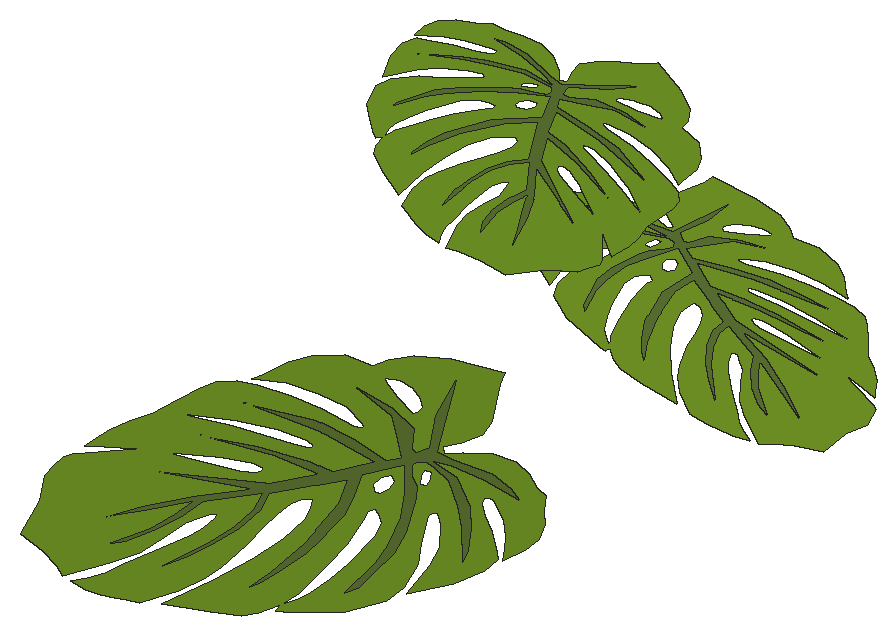
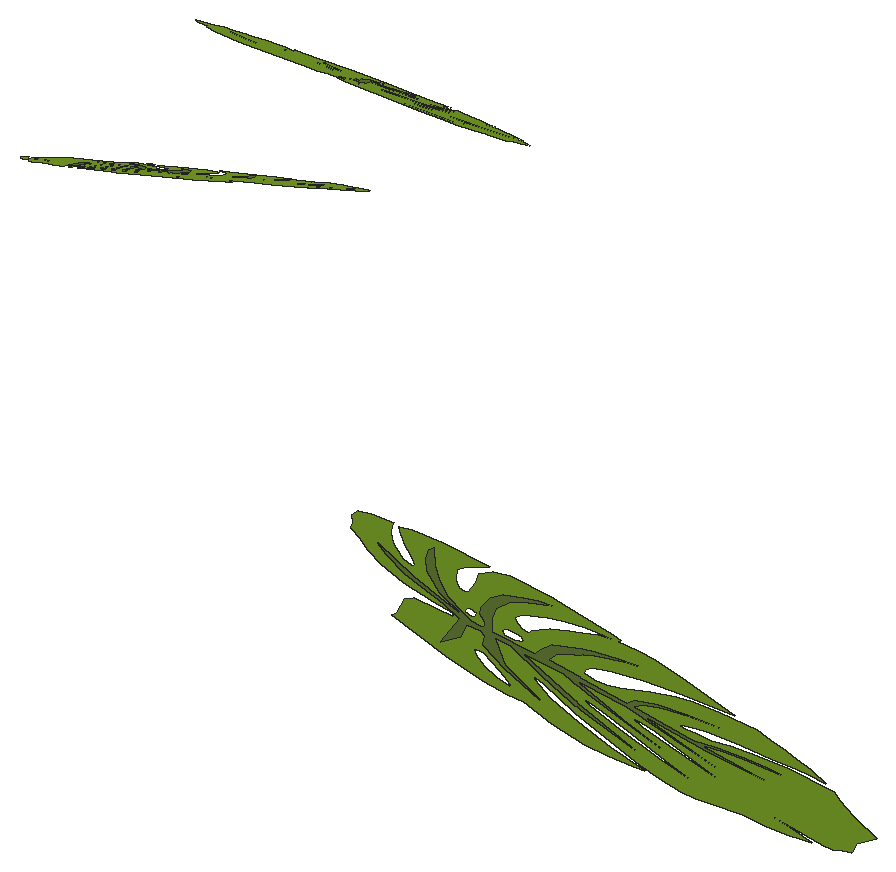
# SketchUp Ruby script. Lengths in inches.
U = 1.inch
M = Sketchup.active_model
def pt(a) = Geom::Point3d.new(a.map { |v| v * U })
def face(e, loops, mat)
  f = e.add_face(loops[0].map { |a| pt(a) })
  loops[1..].each { |l| e.add_face(l.map { |a| pt(a) }).erase! }
  f.material = f.back_material = mat if mat
  f
end
# faces: each face lists its corners as indices into pts; further lists are holes
def faces(e, pts, list, mat = nil) = list.each { |f| face(e, (f[0].is_a?(Array) ? f : [f]).map { |l| l.map { |i| pts[i] } }, mat) }
# xy, xz, yz: faces in a plane at the given z, y or x. An outline is a flat list of corners, or four numbers for a rectangle; further outlines are holes
def ring(l) = l.size == 4 ? [[l[0], l[1]], [l[2], l[1]], [l[2], l[3]], [l[0], l[3]]] : l.each_slice(2).to_a
def flat(e, list, mat, &to3) = list.each { |f| face(e, (f[0].is_a?(Array) ? f : [f]).map { |l| ring(l).map { |u, v| to3.(u, v) } }, mat) }
def xy(e, z, list, mat = nil) = flat(e, list, mat) { |x, y| [x, y, z] }
def xz(e, y, list, mat = nil) = flat(e, list, mat) { |x, z| [x, y, z] }
def yz(e, x, list, mat = nil) = flat(e, list, mat) { |y, z| [x, y, z] }
def lines(e, pts, list) = list.each { |a, b| e.add_line(pt(pts[a]), pt(pts[b])) }
# prism: a flat outline (further loops are holes) pulled along v
def prism(e, loops, v, mat = nil)
  f = face(e, loops, mat); d = Geom::Vector3d.new(v.map { |x| x * U })
  f.pushpull(f.normal.samedirection?(d) ? d.length : -d.length)
end
def box(e, o, s, mat = nil) = prism(e, [[o, [o[0] + s[0], o[1], o[2]], [o[0] + s[0], o[1] + s[1], o[2]], [o[0], o[1] + s[1], o[2]]]], [0, 0, s[2]], mat)
def at(x, y, z, deg = 0) = Geom::Transformation.translation(pt([x, y, z])) * Geom::Transformation.rotation(ORIGIN, Z_AXIS, deg.degrees)
def axes(o, x, y, z) = Geom::Transformation.new([*x, 0, *y, 0, *z, 0, *pt(o).to_a, 1])
def part(name) = M.definitions.add(name)
# library, detail: a bought-in or finely detailed component or shape, given as its bounding box
def library(name, o, s) = part(name).tap { |d| box(d.entities, o, s) }
def detail(e, o, s) = box(e.add_group.entities, o, s)
def put(e, d, t, mat = nil) = e.add_instance(d, t).tap { |i| i.material = mat if mat }
def group(e, t, mat = nil) = e.add_group.tap { |g| g.transformation = t; g.material = mat if mat }.entities
root = M.entities
M.materials.add("[0059_DarkOliveGreen]").color = [85, 107, 47]
M.materials.add("[0061_OliveDrab]").color = [107, 142, 35]
p = [[393.515,166.55,16.01],[391.621,166.953,15.703],[389.886,166.712,15.149],[388.907,166.275,14.701],[388.05,165.452,14.111],[387.657,165.18,13.888],
  [389.738,165.127,14.399],[391.87,164.751,14.779],[393.917,164.169,15.045],[395.398,163.449,15.103],[395.678,163.221,15.073],[395.565,163.142,15.008],
  [395.059,163.235,14.92],[392.64,163.969,14.626],[390.5,164.451,14.292],[388.2,164.848,13.878],[386.969,164.965,13.614],[385.915,164.787,13.263],
  [385.338,164.38,12.932],[384.72,163.701,12.468],[384.204,163.077,12.055],[383.945,162.759,11.846],[382.988,162.222,11.358],[382.317,161.608,10.91],
  [381.91,160.98,10.524],[381.643,160.649,10.306],[382.802,160.695,10.625],[384.558,160.756,11.105],[381.423,160.121,10.013],[381.051,159.944,9.838],
  [380.943,159.362,9.548],[380.835,158.779,9.259],[381.64,157.444,8.867],[382.033,155.547,8.117],[383.972,154.783,8.273],[385.329,154.017,8.279],
  [386.085,153.524,8.252],[388.069,154.479,9.191],[389.148,155.225,9.804],[389.899,156.293,10.477],[390.364,157.049,10.935],[390.895,157.416,11.237],
  [391.33,157.717,11.484],[391.623,157.715,11.558],[391.72,157.513,11.493],[391.495,156.919,11.168],[391.112,156.415,10.843],[389.906,155.376,10.067],
  [388.806,154.507,9.394],[388.202,153.956,8.991],[387.495,153.594,8.646],[386.743,153.326,8.333],[387.915,152.935,8.459],[388.914,152.752,8.634],
  [389.808,152.654,8.82],[390.521,152.61,8.984],[391.356,152.509,9.153],[392.894,153.362,9.932],[393.718,154.174,10.508],[394.098,154.884,10.925],
  [394.527,156.206,11.628],[394.651,157.214,12.113],[394.834,158.068,12.543],[395.087,158.703,12.893],[395.525,159.006,13.142],[396.115,159.025,13.302],
  [396.371,158.546,13.153],[396.522,157.893,12.899],[396.228,156.747,12.309],[395.482,155.514,11.564],[394.31,154.151,10.65],[392.512,152.612,9.497],
  [395.512,152.442,10.193],[397.291,152.418,10.64],[398.07,152.66,10.949],[398.884,153.223,11.411],[399.355,153.912,11.841],[399.538,154.843,12.306],
  [399.671,155.635,12.696],[399.825,156.804,13.26],[399.725,157.669,13.623],[399.637,158.345,13.904],[399.522,158.676,14.022],[399.796,158.865,14.178],
  [400.214,158.662,14.194],[400.74,158.164,14.106],[400.997,157.377,13.819],[400.778,155.789,13.05],[400.447,154.855,12.546],[400.001,154.022,12.057],
  [399.579,153.638,11.776],[398.891,152.873,11.256],[399.383,152.844,11.369],[401.112,153.032,11.899],[402.65,153.233,12.385],[404.401,154.005,13.182],
  [404.726,154.816,13.629],[404.479,156.113,14.148],[403.75,157.251,14.471],[403.221,158.293,14.803],[402.947,158.749,14.937],[402.999,159.006,15.065],
  [403.309,158.976,15.132],[403.963,158.449,15.064],[404.872,157.174,14.725],[405.141,156.141,14.331],[405.128,154.49,13.587],[407.202,155.32,14.493],
  [408.289,156.159,15.149],[408.469,156.863,15.511],[408.12,157.226,15.585],[406.972,158.32,15.78],[405.916,159.13,15.872],[405.25,159.767,15.986],
  [405.171,160.022,16.08],[405.46,160.102,16.19],[405.745,159.963,16.202],[407.14,158.945,16.104],[407.937,158.124,15.941],[408.454,157.395,15.746],
  [408.807,156.842,15.589],[409.568,157.522,16.09],[409.798,158.157,16.434],[409.473,158.978,16.719],[408.798,159.747,16.89],[408.333,160.531,17.122],
  [407.493,160.94,17.09],[406.471,161.618,17.131],[405.281,162.197,17.085],[403.7,162.473,16.802],[402.056,162.391,16.342],[401.102,162.194,16.008],
  [400.746,162.588,16.093],[401.536,162.919,16.445],[402.343,163.477,16.903],[402.289,164.205,17.215],[401.685,165.262,17.534],[401.085,166.231,17.815],
  [400.829,166.916,18.056],[397.377,167.33,17.354],[395.307,167.308,16.811],[394.102,166.955,16.343],[388.315,163.821,13.447],[392.798,163.327,14.379],
  [395.765,162.478,14.762],[398.293,161.543,14.993],[399.024,161.792,15.293],[398.016,162.733,15.455],[396.686,163.985,15.675],[393.653,165.243,15.459],
  [396.378,164.383,15.774],[398.405,163.397,15.854],[399.194,162.284,15.557],[399.5625,162.105,15.572],[400.09,162.469,15.871],[399.041,164.227,16.39],
  [398.568,166.217,17.161],[400.642,162.264,15.921],[401.859,161.9375,16.087],[404.472,161.419,16.527],[406.107,160.741,16.644],[407.054,160.154,16.624],
  [404.314,161.067,16.329],[402.051,161.601,15.986],[400.784,161.768,15.735],[402.807,161.018,15.919],[404.715,159.543,15.748],[405.725,158.363,15.478],
  [406.509,157.147,15.135],[406.746,156.536,14.921],[405.165,158.418,15.359],[404.047,159.536,15.573],[402.534,160.767,15.736],[401.22,161.406,15.685],
  [400.481,161.67,15.613],[400.022,161.607,15.466],[399.92,161.404,15.349],[400.363,160.858,15.218],[401.075,160.312,15.156],[401.547,159.665,14.987],
  [402.455,157.793,14.381],[402.744,156.595,13.918],[402.48,155.474,13.347],[402.307,154.565,12.894],[401.81,154.222,12.612],[402.167,155.974,13.491],
  [402.056,156.965,13.907],[401.542,158.53,14.477],[400.685,159.911,14.876],[399.503,161.423,15.25],[397.644,160.635,14.418],[398.089,159.468,14.009],
  [398.453,158.368,13.609],[398.103,156.086,12.495],[397.45,154.957,11.82],[396.878,154.202,11.334],[396.368,153.849,11.044],[396.982,154.918,11.682],
  [397.528,156.678,12.613],[397.698,158.932,13.668],[397.135,160.283,14.129],[393.571,159.076,12.67],[393.833,158.168,12.33],[393.469,157.058,11.738],
  [392.683,155.991,11.057],[391.839,155.187,10.479],[390.564,154.306,9.756],[392.367,156.132,11.039],[393.098,157.188,11.701],[393.338,158.173,12.205],
  [393.153,159.063,12.557],[390.375,158.297,11.498],[389.872,157.318,10.929],[389.01,156.443,10.315],[387.974,155.727,9.727],[386.963,155.411,9.325],
  [388.698,156.611,10.31],[389.388,157.511,10.891],[389.792,158.233,11.319],[387.64,157.49,10.432],[386.48,157.101,9.959],[385.01,156.543,9.33],
  [385.201,156.643,9.424],[387.37,157.721,10.466],[389.579,158.578,11.42],[392.216,159.228,12.39],[385.985,159.668,10.983],[393.086,159.662,12.808],
  [395.203,160.432,13.699],[392.152,161.128,13.226],[387.211,161.84,12.274],[390.851,161.584,13.096],[394.21,161.061,13.725],[395.982,160.635,13.99],
  [397.748,161.39,14.784],[393.908,162.613,14.344],[391.157,162.613,13.636],[393.216,162.196,13.979],[393.723,161.977,14.011],[393.838,161.823,13.972],
  [393.603,161.76,13.883],[392.78,161.884,13.727],[390.817,162.189,13.358],[388.65,162.517,12.948],[386.369,162.769,12.474],[385.295,162.901,12.257],
  [388.539,162.864,13.075],[391.406,160.672,12.829],[392.14,160.473,12.929],[392.186,160.246,12.839],[391.862,160.122,12.7],[391.134,160.103,12.504],
  [390.564,160.183,12.393],[388.274,160.477,11.936],[386.154,160.757,11.515],[389.403,160.797,12.37],[395.594,165.94,16.271],[396.581,165.594,16.37],
  [397.487,165.036,16.353],[398.004,164.545,16.265],[397.956,164.281,16.135],[397.718,164.198,16.036],[396.166,165.017,16.004],[394.946,165.745,16.017],
  [394.715,165.957,16.053],[399.096,159.73,14.386],[398.68,160.133,14.459],[398.773,160.622,14.703],[399.228,160.777,14.89],[399.679,160.441,14.855],
  [399.758,160.018,14.685],[399.483,159.7,14.472],[401.206,161.172,15.576],[401.524,160.736,15.462],[401.537,160.41,15.319],[401.142,160.424,15.224],
  [400.808,160.896,15.35],[400.772,161.242,15.496],[419.861,163.919,33.007],[421.111,164.185,32.805],[422.257,164.026,32.439],[422.903,163.738,32.143],
  [423.468,163.195,31.754],[423.727,163.015,31.607],[422.354,162.98,31.945],[420.947,162.732,32.195],[419.596,162.348,32.371],[418.619,161.872,32.409],
  [418.434,161.722,32.389],[418.508,161.67,32.346],[418.842,161.731,32.288],[420.439,162.216,32.094],[421.851,162.534,31.874],[423.369,162.796,31.601],
  [424.181,162.874,31.426],[424.877,162.756,31.194],[425.258,162.487,30.976],[425.666,162.039,30.67],[426.007,161.627,30.397],[426.177,161.417,30.259],
  [426.809,161.063,29.9375],[427.252,160.657,29.642],[427.521,160.243,29.387],[427.697,160.025,29.243],[426.932,160.055,29.454],[425.773,160.095,29.77],
  [427.842,159.676,29.049],[428.087,159.559,28.934],[428.159,159.175,28.743],[428.23,158.791,28.552],[427.699,157.91,28.293],[427.439,156.658,27.798],
  [426.16,156.153,27.901],[425.264,155.648,27.905],[424.765,155.323,27.888],[423.456,155.952,28.507],[422.743,156.445,28.912],[422.248,157.15,29.356],
  [421.941,157.649,29.658],[421.59,157.891,29.857],[421.303,158.089,30.02],[421.11,158.088,30.069],[421.046,157.955,30.026],[421.195,157.563,29.812],
  [421.447,157.23,29.598],[422.243,156.545,29.085],[422.969,155.971,28.641],[423.368,155.607,28.375],[423.835,155.369,28.148],[424.331,155.192,27.941],
  [423.557,154.933,28.024],[422.898,154.8125,28.139],[422.308,154.748,28.262],[421.838,154.719,28.37],[421.286,154.652,28.482],[420.271,155.215,28.996],
  [419.727,155.751,29.376],[419.477,156.22,29.651],[419.193,157.092,30.116],[419.111,157.758,30.436],[418.991,158.321,30.719],[418.824,158.741,30.951],
  [418.535,158.94,31.115],[418.145,158.953,31.22],[417.976,158.637,31.122],[417.876,158.205,30.954],[418.071,157.449,30.565],[418.563,156.636,30.073],
  [419.336,155.736,29.47],[420.524,154.721,28.709],[418.543,154.608,29.168],[417.369,154.592,29.463],[416.855,154.752,29.667],[416.318,155.124,29.972],
  [416.007,155.578,30.256],[415.886,156.193,30.563],[415.798,156.715,30.82],[415.697,157.487,31.193],[415.763,158.058,31.432],[415.821,158.504,31.617],
  [415.897,158.722,31.696],[415.716,158.847,31.798],[415.44,158.713,31.809],[415.093,158.384,31.751],[414.923,157.865,31.562],[415.068,156.817,31.054],
  [415.286,156.201,30.721],[415.581,155.651,30.398],[415.859,155.397,30.213],[416.313,154.893,29.87],[415.989,154.873,29.945],[414.847,154.998,30.294],
  [413.832,155.13,30.615],[412.677,155.64,31.141],[412.462,156.175,31.436],[412.625,157.031,31.779],[413.106,157.782,31.992],[413.456,158.47,32.211],
  [413.636,158.771,32.299],[413.602,158.941,32.384],[413.398,158.921,32.428],[412.966,158.573,32.383],[412.365,157.731,32.16],[412.188,157.049,31.899],
  [412.196,155.96,31.408],[410.828,156.507,32.006],[410.11,157.061,32.439],[409.992,157.526,32.679],[410.222,157.766,32.727],[410.98,158.488,32.856],
  [411.677,159.022,32.916],[412.116,159.443,32.992],[412.168,159.611,33.054],[411.978,159.664,33.127],[411.789,159.572,33.134],[410.869,158.9,33.07],
  [410.343,158.359,32.962],[410.002,157.877,32.833],[409.768,157.512,32.73],[409.267,157.961,33.06],[409.115,158.38,33.287],[409.329,158.922,33.476],
  [409.775,159.43,33.589],[410.081,159.947,33.742],[410.636,160.217,33.72],[411.31,160.664,33.748],[412.096,161.046,33.717],[413.139,161.229,33.53],
  [414.225,161.175,33.226],[414.854,161.044,33.006],[415.089,161.305,33.0625],[414.567,161.523,33.295],[414.035,161.891,33.597],[414.071,162.371,33.803],
  [414.469,163.069,34.014],[414.865,163.709,34.199],[415.034,164.161,34.358],[417.312,164.434,33.895],[418.679,164.419,33.536],[419.474,164.187,33.227],
  [423.294,162.118,31.316],[420.335,161.792,31.931],[418.376,161.232,32.184],[416.708,160.615,32.336],[416.225,160.779,32.534],[416.891,161.4,32.641],
  [417.768,162.226,32.786],[419.77,163.057,32.644],[417.972,162.489,32.852],[416.634,161.838,32.904],[416.113,161.104,32.709],[415.87,160.986,32.718],
  [415.522,161.226,32.916],[416.214,162.386,33.258],[416.527,163.699,33.767],[415.158,161.091,32.949],[414.354,160.875,33.059],[412.63,160.533,33.349],
  [411.55,160.086,33.426],[410.926,159.698,33.413],[412.734,160.3,33.218],[414.228,160.653,32.992],[415.064,160.763,32.826],[413.729,160.269,32.947],
  [412.469,159.295,32.835],[411.802,158.516,32.657],[411.285,157.713,32.43],[411.129,157.31,32.289],[412.172,158.552,32.578],[412.91,159.29,32.719],
  [413.909,160.103,32.827],[414.776,160.525,32.793],[415.263,160.699,32.745],[415.567,160.657,32.649],[415.634,160.523,32.571],[415.342,160.163,32.485],
  [414.871,159.802,32.444],[414.56,159.375,32.333],[413.961,158.14,31.932],[413.77,157.349,31.627],[413.944,156.609,31.25],[414.059,156.009,30.951],
  [414.386,155.783,30.765],[414.151,156.94,31.345],[414.224,157.593,31.619],[414.563,158.626,31.996],[415.129,159.538,32.259],[415.909,160.536,32.506],
  [417.136,160.016,31.957],[416.842,159.245,31.687],[416.602,158.519,31.423],[416.833,157.013,30.6875],[417.264,156.268,30.242],[417.642,155.769,29.921],
  [417.978,155.537,29.73],[417.573,156.242,30.151],[417.213,157.404,30.765],[417.1,158.891,31.462],[417.472,159.784,31.766],[419.824,158.987,30.803],
  [419.652,158.387,30.579],[419.892,157.655,30.188],[420.41,156.951,29.739],[420.967,156.42,29.357],[421.809,155.838,28.88],[420.619,157.043,29.727],
  [420.137,157.741,30.164],[419.978,158.39,30.496],[420.1,158.978,30.729],[421.934,158.472,30.03],[422.265,157.826,29.654],[422.835,157.249,29.249],
  [423.518,156.777,28.861],[424.185,156.568,28.596],[423.04,157.36,29.246],[422.585,157.953,29.629],[422.318,158.43,29.912],[423.739,157.94,29.326],
  [424.504,157.683,29.014],[425.475,157.315,28.599],[425.348,157.381,28.661],[423.917,158.092,29.349],[422.459,158.658,29.978],[420.719,159.087,30.618],
  [424.831,159.377,29.69],[420.145,159.373,30.894],[418.747,159.881,31.482],[420.761,160.341,31.17],[424.022,160.811,30.542],[421.62,160.642,31.084],
  [419.402,160.296,31.5],[418.233,160.016,31.675],[417.068,160.514,32.198],[419.602,161.321,31.908],[421.418,161.321,31.441],[420.059,161.046,31.667],
  [419.724,160.901,31.689],[419.648,160.799,31.662],[419.804,160.758,31.604],[420.347,160.84,31.501],[421.642,161.041,31.258],[423.072,161.257,30.986],
  [424.578,161.424,30.674],[425.287,161.511,30.53],[423.146,161.486,31.07],[421.253,160.04,30.908],[420.769,159.908,30.974],[420.738,159.759,30.915],
  [420.952,159.677,30.823],[421.433,159.664,30.694],[421.809,159.718,30.621],[423.321,159.911,30.319],[424.72,160.096,30.041],[422.575,160.123,30.605],
  [418.489,163.517,33.18],[417.838,163.289,33.245],[417.24,162.92,33.234],[416.899,162.596,33.176],[416.93,162.422,33.09],[417.088,162.367,33.025],
  [418.112,162.908,33.004],[418.917,163.388,33.012],[419.07,163.528,33.036],[416.178,159.418,31.936],[416.453,159.684,31.984],[416.391,160.007,32.145],
  [416.091,160.109,32.268],[415.793,159.887,32.245],[415.741,159.608,32.133],[415.922,159.399,31.993],[414.785,160.37,32.721],[414.575,160.082,32.646],
  [414.567,159.867,32.552],[414.827,159.876,32.489],[415.048,160.188,32.572],[415.072,160.416,32.668],[410.264,159.724,39.543],[409.777,159.635,39.486],
  [409.493,159.982,39.707],[408.791,160.461,40.01],[407.829,160.755,40.197],[406.803,160.803,40.228],[405.774,160.76,40.2],[405.049,160.794,40.222],
  [404.195,160.553,40.069],[403.253,160.375,39.956],[402.433,160.078,39.768],[402.024,159.72,39.541],[401.826,159.2,39.21],[402.44,159.363,39.314],
  [403.276,159.565,39.442],[404.316,159.735,39.55],[405.794,159.837,39.614],[406.041,159.825,39.607],[406.111,159.711,39.534],[405.867,159.613,39.472],
  [405.037,159.494,39.397],[403.885,159.398,39.336],[402.459,159.195,39.207],[402.001,159.119,39.159],[401.512,158.742,38.92],[401.336,158.06,38.486],
  [401.629,157.117,37.889],[402.966,157.891,38.38],[403.933,158.302,38.64],[405.394,158.653,38.863],[406.129,158.724,38.908],[406.298,158.655,38.864],
  [406.113,158.521,38.78],[405.614,158.382,38.691],[404.519,158.037,38.472],[403.252,157.701,38.259],[402.082,157.162,37.917],[401.574,156.696,37.621],
  [401.763,155.867,37.095],[402.317,155.362,36.775],[402.971,154.811,36.425],[403.224,154.693,36.35],[403.512,154.855,36.453],[403.525,155.234,36.694],
  [403.641,155.526,36.879],[404.111,156.035,37.202],[404.716,156.559,37.534],[405.906,157.359,38.042],[406.666,157.657,38.231],[407.317,157.749,38.289],
  [407.678,157.732,38.279],[407.652,157.57,38.176],[407.329,157.447,38.098],[406.738,157.155,37.912],[405.987,156.778,37.673],[405.107,156.191,37.301],
  [404.525,155.786,37.043],[403.853,155.302,36.737],[403.434,154.374,36.148],[403.6,154.053,35.944],[404.45,153.588,35.648],[405.989,152.864,35.189],
  [406.402,154.064,35.951],[406.964,155.014,36.553],[407.619,155.788,37.045],[408.414,156.402,37.434],[409.016,156.666,37.602],[409.525,156.822,37.701],
  [409.786,156.655,37.595],[409.744,156.396,37.431],[409.345,156.032,37.2],[408.735,155.585,36.916],[407.973,155.081,36.596],[407.097,154.349,36.131],
  [406.696,153.916,35.857],[406.421,153.316,35.476],[406.444,152.507,34.962],[406.916,152.33,34.85],[407.284,152.16,34.742],[407.782,151.966,34.62],
  [408.396,151.784,34.504],[409.262,151.653,34.421],[409.129,151.98,34.628],[409.093,152.338,34.855],[409.26,152.757,35.121],[409.454,153.457,35.565],
  [409.737,154.264,36.078],[409.968,154.602,36.292],[410.347,154.94,36.506],[410.556,155.008,36.55],[410.694,154.93,36.5],[410.652,154.674,36.338],
  [410.601,154.36,36.139],[410.204,153.883,35.836],[409.685,153.183,35.392],[409.581,152.546,34.987],[409.73,151.57,34.368],[410.484,151.597,34.385],
  [411.741,151.592,34.382],[413.268,151.43,34.279],[414.995,152.209,34.774],[416.457,152.617,35.032],[416.88,152.918,35.223],[417.304,153.219,35.414],
  [417.274,153.401,35.53],[416.328,154.536,36.25],[417.098,154.038,35.934],[417.601,153.706,35.723],[417.746,153.932,35.867],[418.067,154.334,36.122],
  [418.254,154.8,36.418],[418.244,155.307,36.739],[418.382,155.525,36.878],[418.648,155.954,37.15],[418.913,156.436,37.456],[418.975,156.781,37.675],
  [418.628,157.146,37.907],[417.958,157.42,38.081],[416.561,157.851,38.354],[415.171,158.199,38.575],[413.444,158.503,38.768],[413.133,158.596,38.827],
  [413.144,158.663,38.869],[413.46,158.694,38.889],[414.738,158.634,38.851],[416.166,158.358,38.676],[417.467,157.962,38.425],[418.482,157.43,38.087],
  [418.519,157.662,38.234],[418.79,158.276,38.624],[418.688,158.742,38.919],[418.074,159.318,39.285],[416.862,159.637,39.488],[416.919,159.984,39.708],
  [416.643,160.471,40.017],[415.695,161.035,40.375],[413.747,161.766,40.839],[413.07,161.514,40.679],[412.001,161.223,40.494],[410.859,160.891,40.284],
  [410.242,160.566,40.077],[410.165,160.09,39.775],[411.458,156.308,37.375],[414.776,154.41,36.17],[411.511,155.873,37.099],[412.212,154.864,36.458],
  [412.546,153.872,35.829],[412.681,152.789,35.141],[412.688,152.691,35.079],[412.457,153.345,35.494],[412.232,153.837,35.806],[411.832,154.76,36.392],
  [411.433,154.314,36.11],[411.022,153.71,35.726],[410.856,152.685,35.076],[410.642,153.104,35.341],[410.741,153.715,35.729],[411.05,154.354,36.135],
  [411.612,154.945,36.51],[410.939,156.046,37.209],[410.128,155.68,36.976],[409.439,155.157,36.644],[408.921,154.468,36.207],[408.276,153.134,35.36],
  [408.398,153.886,35.838],[408.658,154.487,36.219],[409.16,155.195,36.669],[409.893,155.81,37.059],[410.754,156.164,37.284],[410.074,157.682,38.247],
  [408.711,157.202,37.942],[406.957,156.104,37.246],[405.779,155.137,36.632],[405.195,154.473,36.211],[405.244,154.775,36.402],[405.592,155.28,36.723],
  [406.206,155.982,37.168],[407.9,157.141,37.903],[408.965,157.556,38.167],[410.123,157.982,38.4375],[409.896,158.847,38.986],[408.114,158.458,38.739],
  [406.59,158.043,38.476],[405.077,157.45,38.1],[404.219,157.018,37.825],[402.959,156.104,37.246],[403.007,156.397,37.432],[403.665,156.868,37.73],
  [404.455,157.462,38.107],[405.564,157.943,38.413],[407.511,158.574,38.813],[408.258,158.749,38.924],[409.035,158.814,38.965],[409.685,158.95,39.052],
  [409.803,159.072,39.129],[409.64,159.224,39.226],[409.081,159.299,39.273],[407.948,159.353,39.307],[406.239,159.183,39.199],[404.808,158.96,39.058],
  [402.539,158.505,38.769],[403.146,158.727,38.91],[404.502,159.085,39.137],[405.934,159.365,39.315],[408.025,159.543,39.428],[409.579,159.351,39.306],
  [408.852,159.612,39.472],[407.361,159.969,39.698],[405.339,160.276,39.893],[406.259,160.297,39.906],[407.574,160.176,39.829],[409.215,159.718,39.539],
  [410.049,159.545,39.429],[414.233,160.834,40.247],[412.393,160.032,39.738],[410.474,159.493,39.396],[410.423,159.181,39.199],[410.741,159.166,39.189],
  [412.014,159.475,39.385],[413.763,159.392,39.332],[415.734,159.064,39.124],[413.295,159.289,39.267],[411.656,159.061,39.122],[410.42,158.892,39.015],
  [410.558,158.579,38.816],[412.499,158.339,38.664],[414.574,157.941,38.411],[417.069,156.972,37.796],[413.475,157.905,38.389],[410.688,158.362,38.679],
  [410.898,157.537,38.155],[412.071,157.262,37.98],[414.065,156.607,37.565],[415.972,155.752,37.022],[413.087,156.742,37.651],[411.096,157.234,37.963],
  [414.759,157.169,37.921],[415.675,156.794,37.683],[416.185,156.585,37.551],[417.729,155.734,37.011],[417.121,155.96,37.154],[415.851,156.453,37.467],
  [414.573,156.88,37.738],[413.409,157.263,37.981],[412.924,157.425,38.084],[412.865,157.518,38.143],[413.044,157.559,38.169],[413.459,157.525,38.147],
  [413.582,156.091,37.237],[413.846,155.969,37.16],[414.1,155.852,37.086],[415.584,154.963,36.522],[414.367,155.4,36.799],[413.059,155.876,37.101],
  [412.727,155.991,37.174],[412.403,156.195,37.303],[412.353,156.34,37.395],[412.559,156.433,37.454],[413.063,156.33,37.389],[414.216,160.003,39.72],
  [414.654,160.012,39.726],[415.396,159.909,39.66],[415.82,159.682,39.516],[415.54,159.645,39.493],[414.378,159.632,39.484],[412.987,159.665,39.505],
  [412.944,159.767,39.57],[413.136,159.903,39.656],[413.777,159.994,39.714],[409.585,158.278,38.625],[409.23,158.025,38.465],[408.708,157.948,38.416],
  [408.503,158.038,38.473],[408.633,158.26,38.614],[409.015,158.436,38.725],[409.499,158.472,38.748],[408.54,159.102,39.148],[408.897,159.186,39.201],
  [409.156,159.103,39.148],[408.859,158.951,39.052],[408.318,158.82,38.969],[408.122,158.919,39.032],[408.393,159.067,39.126],[410.527,157.975,24.504],
  [410.532,157.973,24.503],[408.63,158.258,38.613]]
faces(root,p,[[[0,1,2,3,4,5,6,7,8,9,10,11,12,13,14,15,16,17,18,19,20,21,22,23,24,25,26,27,28,29,30,31,32,33,34,35,36,37,38,39,40,41,42,43,44,45,46,47,48,49,50,51,52,53,54,55,56,57,58,59,60,61,62,63,64,65,66,67,68,69,70,71,72,73,74,75,76,77,78,79,80,81,82,83,84,85,86,87,88,89,90,75,91,92,93,94,95,96,97,98,99,100,101,102,103,104,105,106,107,108,109,110,111,112,113,114,115,116,117,118,119,120,121,122,123,124,125,126,127,128,129,130,131,132,133,134,135,136,137,138,139,140,141],[142,143,144,145,146,147,148,149,150,151,152,153,154,155,156,157,158,159,160,161,162,163,164,165,166,167,168,169,170,171,172,173,174,175,176,177,178,179,180,181,182,183,184,185,186,187,188,189,190,191,192,193,194,195,196,197,198,199,200,201,202,203,204,205,206,207,208,209,210,211,212,213,214,215,216,217,218,219,220,221,222,223,224,225,226,227,228,229,230,231,232,233,234,235],[236,237,238,239,240,241,242,243,244,245,246],[247,248,249,250,251,252,253,254,255],[256,257,258,259,260,261,262,263,264],[265,266,267,268,269,270,271],[272,273,274,275,276,277]],[[278,279,280,281,282,283,284,285,286,287,288,289,290,291,292,293,294,295,296,297,298,299,300,301,302,303,304,305,306,307,308,309,310,311,312,313,314,315,316,317,318,319,320,321,322,323,324,325,326,327,328,329,330,331,332,333,334,335,336,337,338,339,340,341,342,343,344,345,346,347,348,349,350,351,352,353,354,355,356,357,358,359,360,361,362,363,364,365,366,367,368,353,369,370,371,372,373,374,375,376,377,378,379,380,381,382,383,384,385,386,387,388,389,390,391,392,393,394,395,396,397,398,399,400,401,402,403,404,405,406,407,408,409,410,411,412,413,414,415,416,417,418,419],[420,421,422,423,424,425,426,427,428,429,430,431,432,433,434,435,436,437,438,439,440,441,442,443,444,445,446,447,448,449,450,451,452,453,454,455,456,457,458,459,460,461,462,463,464,465,466,467,468,469,470,471,472,473,474,475,476,477,478,479,480,481,482,483,484,485,486,487,488,489,490,491,492,493,494,495,496,497,498,499,500,501,502,503,504,505,506,507,508,509,510,511,512,513],[514,515,516,517,518,519,520,521,522,523,524],[525,526,527,528,529,530,531,532,533],[534,535,536,537,538,539,540,541,542],[543,544,545,546,547,548,549],[550,551,552,553,554,555]],[[556,557,558,559,560,561,562,563,564,565,566,567,568,569,570,571,572,573,574,575,576,577,578,579,580,581,582,583,584,585,586,587,588,589,590,591,592,593,594,595,596,597,598,599,600,601,602,603,604,605,606,607,608,609,610,611,612,613,598,614,615,616,617,618,619,620,621,622,623,624,625,626,627,628,629,630,631,632,633,634,635,636,637,638,639,640,641,642,643,644,645,646,647,648,649,650,651,652,653,654,655,656,657,658,659,660,661,662,663,664,665,666,667,668,669,670,671,672,673,674,675,676,677,678,679,680,681,682,683,684,685,686,687,688,689,690,691,692,693,694,695,696,697],[698,699,700,701,702,703,704,705,706,707,708,709,710,711,712,713,714,715,716,717,718,719,720,721,722,723,724,725,726,727,728,729,730,731,732,733,734,735,736,737,738,739,740,741,742,743,744,745,746,747,748,749,750,751,752,753,754,755,756,757,758,759,760,761,762,763,764,765,766,767,768,769,770,771,772,773,774,775,776,777,778,779,780,781,782,783,784,785,786,787,788,789,790,791],[792,793,794,795,796,797,798,799,800,801,802,803],[804,805,806,807,808,809,810,811,812,813,814],[815,816,817,818,819,820,821,822,823,824],[825,826,827,828,829,830,831],[832,833,834,835,836,837,838]]],"[0061_OliveDrab]")
faces(root,p,[[143,142,235,234,233,232,231,230,229,228,227,226,225,224,223,222,221,220,219,218,217,216,215,214,213,212,211,210,209,208,207,206,205,204,203,202,201,200,199,198,197,196,195,194,193,192,191,190,189,188,187,186,185,184,183,182,181,180,179,178,177,176,175,174,173,172,171,170,169,168,167,166,165,164,163,162,161,160,159,158,157,156,155,154,153,152,151,150,149,148,147,146,145,144],[421,420,513,512,511,510,509,508,507,506,505,504,503,502,501,500,499,498,497,496,495,494,493,492,491,490,489,488,487,486,485,484,483,482,481,480,479,478,477,476,475,474,473,472,471,470,469,468,467,466,465,464,463,462,461,460,459,458,457,456,455,454,453,452,451,450,449,448,447,446,445,444,443,442,441,440,439,438,437,436,435,434,433,432,431,430,429,428,427,426,425,424,423,422],[699,698,791,790,789,788,787,786,785,784,783,782,781,780,779,778,777,776,775,774,773,772,771,770,769,768,767,766,765,764,763,762,761,760,759,758,757,756,755,754,753,752,751,750,749,748,747,746,745,744,743,742,741,740,739,738,737,736,735,734,733,732,731,730,729,728,727,726,725,724,723,722,721,720,719,718,717,716,715,714,713,712,711,710,709,708,707,706,705,704,703,702,701,700]],"[0059_DarkOliveGreen]")
lines(root,p,[[839,840],[829,841]])
